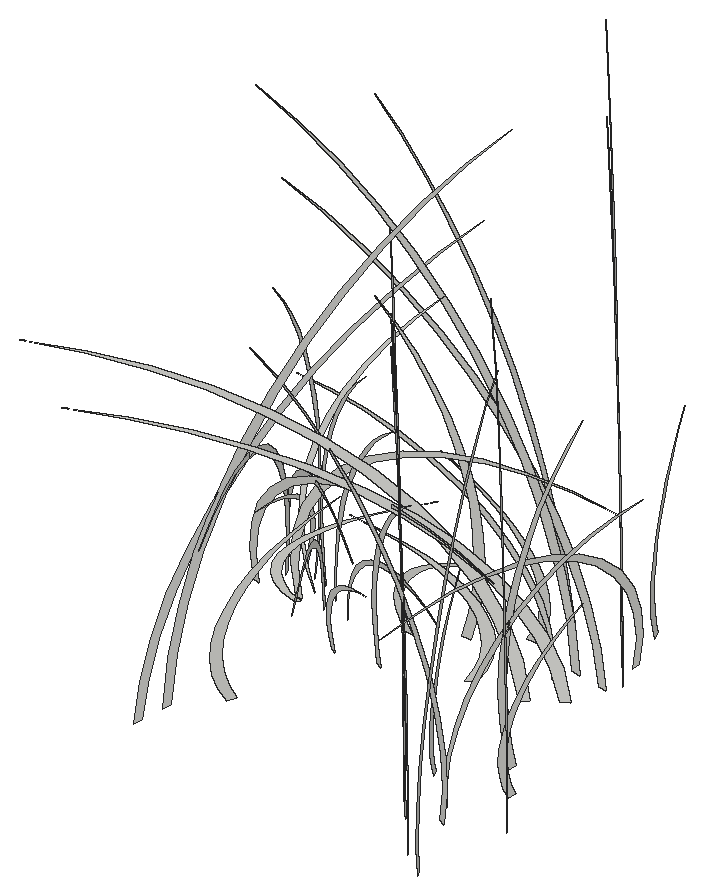
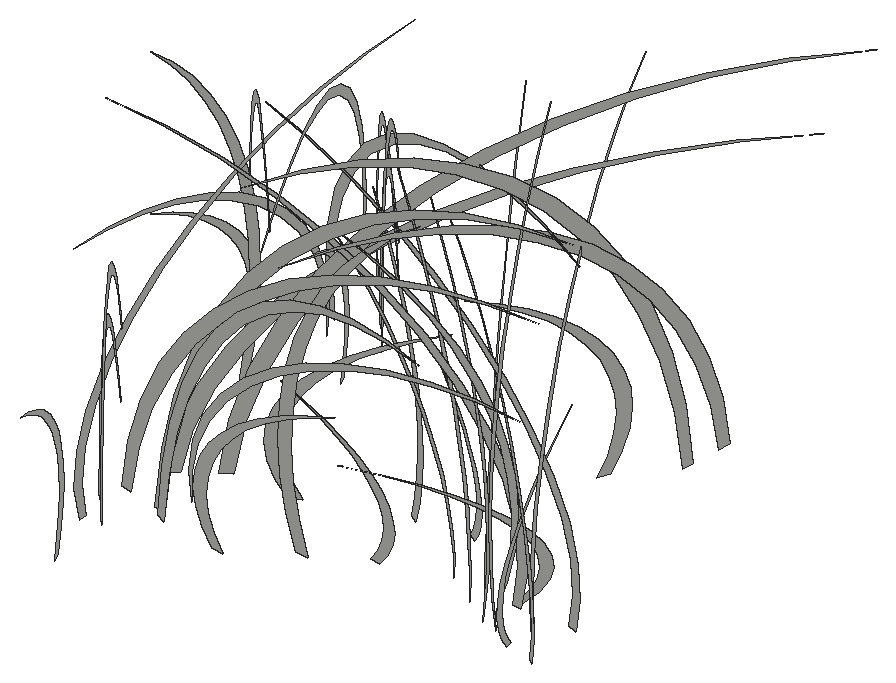
# SketchUp Ruby script. Lengths in inches.
U = 1.inch
M = Sketchup.active_model
def pt(a) = Geom::Point3d.new(a.map { |v| v * U })
def face(e, loops, mat)
  f = e.add_face(loops[0].map { |a| pt(a) })
  loops[1..].each { |l| e.add_face(l.map { |a| pt(a) }).erase! }
  f.material = f.back_material = mat if mat
  f
end
# faces: each face lists its corners as indices into pts; further lists are holes
def faces(e, pts, list, mat = nil) = list.each { |f| face(e, (f[0].is_a?(Array) ? f : [f]).map { |l| l.map { |i| pts[i] } }, mat) }
# xy, xz, yz: faces in a plane at the given z, y or x. An outline is a flat list of corners, or four numbers for a rectangle; further outlines are holes
def ring(l) = l.size == 4 ? [[l[0], l[1]], [l[2], l[1]], [l[2], l[3]], [l[0], l[3]]] : l.each_slice(2).to_a
def flat(e, list, mat, &to3) = list.each { |f| face(e, (f[0].is_a?(Array) ? f : [f]).map { |l| ring(l).map { |u, v| to3.(u, v) } }, mat) }
def xy(e, z, list, mat = nil) = flat(e, list, mat) { |x, y| [x, y, z] }
def xz(e, y, list, mat = nil) = flat(e, list, mat) { |x, z| [x, y, z] }
def yz(e, x, list, mat = nil) = flat(e, list, mat) { |y, z| [x, y, z] }
def lines(e, pts, list) = list.each { |a, b| e.add_line(pt(pts[a]), pt(pts[b])) }
# prism: a flat outline (further loops are holes) pulled along v
def prism(e, loops, v, mat = nil)
  f = face(e, loops, mat); d = Geom::Vector3d.new(v.map { |x| x * U })
  f.pushpull(f.normal.samedirection?(d) ? d.length : -d.length)
end
def box(e, o, s, mat = nil) = prism(e, [[o, [o[0] + s[0], o[1], o[2]], [o[0] + s[0], o[1] + s[1], o[2]], [o[0], o[1] + s[1], o[2]]]], [0, 0, s[2]], mat)
def at(x, y, z, deg = 0) = Geom::Transformation.translation(pt([x, y, z])) * Geom::Transformation.rotation(ORIGIN, Z_AXIS, deg.degrees)
def axes(o, x, y, z) = Geom::Transformation.new([*x, 0, *y, 0, *z, 0, *pt(o).to_a, 1])
def part(name) = M.definitions.add(name)
# library, detail: a bought-in or finely detailed component or shape, given as its bounding box
def library(name, o, s) = part(name).tap { |d| box(d.entities, o, s) }
def detail(e, o, s) = box(e.add_group.entities, o, s)
def put(e, d, t, mat = nil) = e.add_instance(d, t).tap { |i| i.material = mat if mat }
def group(e, t, mat = nil) = e.add_group.tap { |g| g.transformation = t; g.material = mat if mat }.entities
root = M.entities
g1 = group(root,at(61.625,583.2,0.02))
p = [[2.45,-7.42,6.49],[1.99,-6.01,6.08],[1.56,-4.73,5.625],[1.19,-3.6,5.14],[0.87,-2.64,4.62],[0.61,-1.83,4.08],
  [0.4,-1.21,3.52],[0.25,-0.76,2.9375],[0.16,-0.5,2.35],[0.14,-0.42,1.76],[0.18,-0.53,1.16],[0.28,-0.83,0.58],
  [0.43,-1.3125,0],[0.33,-0.99,0],[0.15,-0.44,0.57],[0.03,-0.1,1.16],[-0.02,0.05,1.75],[0.01,-0.02,2.35],
  [0.09,-0.28,2.94],[0.25,-0.76,3.53],[0.47,-1.43,4.1],[0.76,-2.29,4.64],[1.1,-3.33,5.16],[1.5,-4.54,5.65],
  [1.95,-5.91,6.09]]
faces(g1,p,[[0,1,2,3,4,5,6,7,8,9,10,11,12,13,14,15,16,17,18,19,20,21,22,23,24]])
g2 = group(root,at(62.74,582.29,0.02))
p = [[0.26,-0.74,0],[0.12,-0.33,1.62],[0.03,-0.08,3.26],[0,0,4.9],[0.03,-0.08,6.54],[0.11,-0.32,8.18],
  [0.26,-0.73,9.8],[0.46,-1.29,11.4],[0.71,-2.02,12.97],[1.03,-2.89,14.51],[1.39,-3.92,16],[1.8,-5.1,17.45],
  [2.27,-6.41,18.84],[1.83,-5.17,17.43],[1.44,-4.07,15.97],[1.09,-3.09,14.46],[0.8,-2.25,12.93],[0.55,-1.56,11.36],
  [0.35,-1,9.76],[0.21,-0.59,8.15],[0.12,-0.33,6.52],[0.07,-0.21,4.89],[0.08,-0.24,3.25],[0.15,-0.41,1.62]]
faces(g2,p,[[0,1,2,3,4,5,6,7,8,9,10,11,12,13,14,15,16,17,18,19,20,21,22,23]])
g3 = group(root,at(62.67,578.69,0.02))
p = [[6.35,4.55,5.51],[5.14,3.68,5.16],[4.05,2.9,4.78],[3.09,2.21,4.37],[2.26,1.62,3.93],[1.57,1.125,3.47],
  [1.03,0.74,2.99],[0.65,0.47,2.5],[0.43,0.31,2],[0.36,0.26,1.49],[0.46,0.33,0.99],[0.71,0.51,0.49],
  [1.125,0.8,0],[0.85,0.61,0],[0.38,0.27,0.48],[0.08,0.06,0.98],[-0.04,-0.03,1.49],[0.01,0.01,2],
  [0.24,0.17,2.5],[0.65,0.46,3],[1.22,0.875,3.48],[1.96,1.4,3.95],[2.85,2.04,4.39],[3.89,2.78,4.8],
  [5.0625,3.62,5.18]]
faces(g3,p,[[0,1,2,3,4,5,6,7,8,9,10,11,12,13,14,15,16,17,18,19,20,21,22,23,24]])
g4 = group(root,at(63.21,580.03,0.02))
p = [[0.625,0.47,0],[0.28,0.21,1.38],[0.07,0.05,2.77],[0,0,4.16],[0.07,0.05,5.5625],[0.28,0.21,6.95],
  [0.62,0.46,8.33],[1.1,0.82,9.69],[1.71,1.28,11.03],[2.46,1.84,12.33],[3.33,2.49,13.6],[4.33,3.24,14.83],
  [5.45,4.07,16.01],[4.4,3.29,14.8125],[3.46,2.58,13.57],[2.63,1.96,12.3],[1.92,1.43,10.99],[1.32,0.99,9.65],
  [0.85,0.64,8.3],[0.5,0.375,6.93],[0.28,0.21,5.55],[0.18,0.13,4.16],[0.2,0.15,2.77],[0.35,0.26,1.38]]
faces(g4,p,[[0,1,2,3,4,5,6,7,8,9,10,11,12,13,14,15,16,17,18,19,20,21,22,23]])
g5 = group(root,at(65.02,565.47,0.02))
p = [[1.63,20.71,16.73],[1.875,23.84,17.17],[1.64,20.8125,16.64],[1.41,17.89,15.9],[1.1875,15.1,14.96],[0.98,12.48,13.84],
  [0.79,10.06,12.54],[0.62,7.86,11.08],[0.47,5.91,9.48],[0.33,4.23,7.76],[0.22,2.84,5.92],[0.14,1.75,4.01],
  [0.08,0.98,2.02],[0.04,0.54,0],[0,0,0],[0.03,0.36,2.07],[0.09,1.09,4.1],[0.17,2.15,6.07],
  [0.28,3.55,7.94],[0.41,5.27,9.7],[0.57,7.28,11.33],[0.75,9.55,12.79],[0.95,12.07,14.08],[1.16,14.79,15.17],
  [1.39,17.68,16.0625]]
faces(g5,p,[[0,1,2,3,4,5,6,7,8,9,10,11,12,13,14,15,16,17,18,19,20,21,22,23,24]])
g6 = group(root,at(63.16,581.76,0.02))
p = [[0.65,-0.43,0],[0.29,-0.19,1.24],[0.07,-0.05,2.49],[0,0,3.75],[0.07,-0.05,5.01],[0.29,-0.1875,6.26],
  [0.65,-0.43,7.5],[1.15,-0.75,8.73],[1.79,-1.18,9.93],[2.57,-1.6875,11.11],[3.48,-2.29,12.25],[4.52,-2.97,13.36],
  [5.68,-3.74,14.43],[4.59,-3.02,13.35],[3.6,-2.37,12.23],[2.74,-1.8,11.08],[2,-1.3125,9.9],[1.38,-0.91,8.7],
  [0.89,-0.58,7.48],[0.52,-0.34,6.24],[0.29,-0.19,5],[0.18,-0.12,3.74],[0.21,-0.14,2.49],[0.37,-0.24,1.24]]
faces(g6,p,[[0,1,2,3,4,5,6,7,8,9,10,11,12,13,14,15,16,17,18,19,20,21,22,23]])
g7 = group(root,at(65.17,567.4,0.02))
p = [[1.63,20.71,20.75],[1.875,23.84,21.3],[1.64,20.8125,20.63],[1.41,17.89,19.72],[1.1875,15.1,18.55],[0.98,12.48,17.16],
  [0.79,10.06,15.55],[0.62,7.86,13.74],[0.47,5.91,11.76],[0.33,4.23,9.62],[0.22,2.84,7.35],[0.14,1.75,4.97],
  [0.08,0.98,2.51],[0.04,0.54,0],[0,0,0],[0.03,0.36,2.57],[0.09,1.09,5.09],[0.17,2.15,7.53],
  [0.28,3.55,9.85],[0.41,5.27,12.03],[0.57,7.28,14.04],[0.75,9.55,15.86],[0.95,12.07,17.46],[1.16,14.79,18.82],
  [1.39,17.68,19.92]]
faces(g7,p,[[0,1,2,3,4,5,6,7,8,9,10,11,12,13,14,15,16,17,18,19,20,21,22,23,24]])
g8 = group(root,at(61.36,581.64,0.02))
p = [[0.35,-0.68,0],[0.16,-0.3,0],[0,0,1.7],[0.0625,-0.12,3.4],[0.34,-0.66,5.07],[0.83,-1.61,6.67],
  [1.52,-2.93,8.15],[2.39,-4.61,9.48],[3.42,-6.59,10.63],[4.58,-8.84,11.57],[5.85,-11.28,12.27],[7.1875,-13.87,12.71],
  [8.57,-16.53,12.89],[9.96,-19.21,12.81],[8.6,-16.58,12.82],[7.25,-13.98,12.59],[5.95,-11.47,12.1],[4.72,-9.1,11.38],
  [3.59,-6.93,10.4375],[2.6,-5.01,9.3],[1.75,-3.38,7.99],[1.08,-2.09,6.53],[0.6,-1.15,4.97],[0.31,-0.6,3.33],
  [0.23,-0.4375,1.67]]
faces(g8,p,[[0,1,2,3,4,5,6,7,8,9,10,11,12,13,14,15,16,17,18,19,20,21,22,23,24]])
g9 = group(root,at(78.42,582.08,0.02))
p = [[-20.32,4.32,20.75],[-23.39,4.97,21.3],[-20.42,4.34,20.63],[-17.55,3.73,19.72],[-14.82,3.15,18.55],[-12.25,2.6,17.16],
  [-9.87,2.1,15.55],[-7.71,1.64,13.74],[-5.8,1.23,11.76],[-4.15,0.88,9.62],[-2.79,0.59,7.35],[-1.72,0.37,4.97],
  [-0.96,0.21,2.51],[-0.53,0.11,0],[0,0,0],[-0.36,0.08,2.57],[-1.07,0.23,5.09],[-2.11,0.45,7.53],
  [-3.49,0.74,9.85],[-5.17,1.1,12.03],[-7.14,1.52,14.04],[-9.375,1.99,15.86],[-11.84,2.52,17.46],[-14.51,3.08,18.82],
  [-17.35,3.6875,19.92]]
faces(g9,p,[[0,1,2,3,4,5,6,7,8,9,10,11,12,13,14,15,16,17,18,19,20,21,22,23,24]])
g10 = group(root,at(60.26,582.81,0.02))
p = [[0.47,-0.41,0],[0.21,-0.18,0],[0,0,1.2],[0.08,-0.07,2.41],[0.46,-0.4,3.6],[1.12,-0.98,4.74],
  [2.04,-1.79,5.79],[3.2,-2.8125,6.73],[4.58,-4.02,7.55],[6.13,-5.39,8.21],[7.83,-6.875,8.71],[9.62,-8.45,9.03],
  [11.47,-10.08,9.16],[13.33,-11.71,9.09],[11.51,-10.11,9.11],[9.7,-8.52,8.9375],[7.96,-6.99,8.59],[6.31,-5.55,8.08],
  [4.81,-4.22,7.41],[3.48,-3.05,6.6],[2.35,-2.0625,5.67],[1.45,-1.27,4.64],[0.8,-0.7,3.53],[0.41,-0.36,2.37],
  [0.3,-0.27,1.18]]
faces(g10,p,[[0,1,2,3,4,5,6,7,8,9,10,11,12,13,14,15,16,17,18,19,20,21,22,23,24]])
g11 = group(root,at(60.26,582.81,0.02))
p = [[0.47,-0.41,0],[0.21,-0.18,0],[0,0,1.2],[0.08,-0.07,2.41],[0.46,-0.4,3.6],[1.12,-0.98,4.74],
  [2.04,-1.79,5.79],[3.2,-2.8125,6.73],[4.58,-4.02,7.55],[6.13,-5.39,8.21],[7.83,-6.875,8.71],[9.62,-8.45,9.03],
  [11.47,-10.08,9.16],[13.33,-11.71,9.09],[11.51,-10.11,9.11],[9.7,-8.52,8.9375],[7.96,-6.99,8.59],[6.31,-5.55,8.08],
  [4.81,-4.22,7.41],[3.48,-3.05,6.6],[2.35,-2.0625,5.67],[1.45,-1.27,4.64],[0.8,-0.7,3.53],[0.41,-0.36,2.37],
  [0.3,-0.27,1.18]]
faces(g11,p,[[0,1,2,3,4,5,6,7,8,9,10,11,12,13,14,15,16,17,18,19,20,21,22,23,24]])
g12 = group(root,at(77.95,582.5,0.02))
p = [[-18.35,9.75,18.05],[-21.11,11.23,18.53],[-18.43,9.8,17.95],[-15.84,8.42,17.15],[-13.375,7.11,16.14],[-11.05,5.88,14.93],
  [-8.91,4.74,13.53],[-6.96,3.7,11.96],[-5.23,2.78,10.23],[-3.75,1.99,8.37],[-2.51,1.34,6.39],[-1.55,0.83,4.32],
  [-0.87,0.46,2.18],[-0.48,0.25,0],[0,0,0],[-0.32,0.17,2.23],[-0.96,0.51,4.43],[-1.91,1.01,6.55],
  [-3.15,1.67,8.57],[-4.67,2.48,10.47],[-6.45,3.43,12.22],[-8.46,4.5,13.8],[-10.6875,5.68,15.1875],[-13.1,6.97,16.37],
  [-15.66,8.33,17.33]]
faces(g12,p,[[0,1,2,3,4,5,6,7,8,9,10,11,12,13,14,15,16,17,18,19,20,21,22,23,24]])
g13 = group(root,at(66.72,568.99,0.02))
p = [[2.34,6.79,9.0625],[1.91,5.55,8.49],[1.52,4.43,7.85],[1.18,3.44,7.18],[0.89,2.58,6.45],[0.65,1.88,5.7],
  [0.46,1.33,4.91],[0.32,0.93,4.1],[0.24,0.7,3.28],[0.22,0.64,2.45],[0.25,0.74,1.625],[0.34,1,0.8],
  [0.49,1.42,0],[0.3,0.875,0],[0.14,0.4,0.81],[0.04,0.11,1.65],[0,0,2.49],[0.03,0.07,3.34],
  [0.11,0.33,4.17],[0.27,0.77,4.99],[0.48,1.38,5.79],[0.75,2.17,6.54],[1.07,3.11,7.26],[1.45,4.2,7.92],
  [1.87,5.43,8.52]]
faces(g13,p,[[0,1,2,3,4,5,6,7,8,9,10,11,12,13,14,15,16,17,18,19,20,21,22,23,24]])
g14 = group(root,at(78.15,578.71,0.02))
p = [[-17.04,-11.89,18.05],[-19.61,-13.68,18.53],[-17.12,-11.94,17.95],[-14.72,-10.27,17.15],[-12.42,-8.67,16.14],[-10.27,-7.16,14.93],
  [-8.28,-5.77,13.53],[-6.47,-4.51,11.96],[-4.86,-3.39,10.23],[-3.48,-2.43,8.37],[-2.34,-1.63,6.39],[-1.44,-1.01,4.32],
  [-0.81,-0.5625,2.18],[-0.44,-0.31,0],[0,0,0],[-0.3,-0.21,2.23],[-0.89,-0.62,4.43],[-1.77,-1.24,6.55],
  [-2.92,-2.04,8.57],[-4.33,-3.02,10.47],[-5.99,-4.18,12.22],[-7.86,-5.48,13.8],[-9.93,-6.93,15.1875],[-12.17,-8.49,16.37],
  [-14.55,-10.15,17.33]]
faces(g14,p,[[0,1,2,3,4,5,6,7,8,9,10,11,12,13,14,15,16,17,18,19,20,21,22,23,24]])
g15 = group(root,at(80.31,581.68,0.02))
p = [[-20.32,4.32,16.73],[-23.39,4.97,17.17],[-20.42,4.34,16.64],[-17.55,3.73,15.9],[-14.82,3.15,14.96],[-12.25,2.6,13.84],
  [-9.87,2.1,12.54],[-7.71,1.64,11.08],[-5.8,1.23,9.48],[-4.15,0.88,7.76],[-2.79,0.59,5.92],[-1.72,0.37,4.01],
  [-0.96,0.21,2.02],[-0.53,0.11,0],[0,0,0],[-0.36,0.08,2.07],[-1.07,0.23,4.1],[-2.11,0.45,6.07],
  [-3.49,0.74,7.94],[-5.17,1.1,9.7],[-7.14,1.52,11.33],[-9.375,1.99,12.79],[-11.84,2.52,14.08],[-14.51,3.08,15.17],
  [-17.35,3.6875,16.0625]]
faces(g15,p,[[0,1,2,3,4,5,6,7,8,9,10,11,12,13,14,15,16,17,18,19,20,21,22,23,24]])
g16 = group(root,at(64.98,580.56,0.02))
p = [[7.3,-4.8,13.72],[6.14,-4.04,12.71],[5.07,-3.33,11.66],[4.1,-2.69,10.58],[3.22,-2.12,9.48],[2.46,-1.61,8.34],
  [1.79,-1.18,7.19],[1.23,-0.8125,6.02],[0.79,-0.52,4.83],[0.45,-0.29,3.63],[0.22,-0.14,2.43],[0.1,-0.07,1.21],
  [0.1,-0.0625,0],[0,0,1.22],[0.04,-0.02,2.44],[0.2,-0.13,3.66],[0.5,-0.33,4.87],[0.92,-0.61,6.07],
  [1.47,-0.97,7.25],[2.15,-1.41,8.41],[2.95,-1.9375,9.54],[3.87,-2.54,10.64],[4.9,-3.22,11.71],[6.05,-3.98,12.73]]
faces(g16,p,[[0,1,2,3,4,5,6,7,8,9,10,11,12,13,14,15,16,17,18,19,20,21,22,23]])
g17 = group(root,at(77.73,581,0.02))
p = [[-16.72,1.64,9.9],[-14.47,1.42,9.83],[-12.26,1.2,9.59],[-10.125,0.99,9.18],[-8.11,0.8,8.61],[-6.26,0.61,7.88],
  [-4.6,0.45,7.02],[-3.17,0.31,6.03],[-1.98,0.19,4.95],[-1.08,0.11,3.78],[-0.46,0.05,2.55],[-0.15,0.01,1.28],
  [-0.15,0.01,0],[0,0,1.3],[-0.2,0.02,2.61],[-0.73,0.07,3.875],[-1.6,0.16,5.09],[-2.77,0.27,6.21],
  [-4.23,0.41,7.22],[-5.93,0.58,8.1],[-7.85,0.77,8.82],[-9.93,0.97,9.37],[-12.14,1.19,9.74],[-14.42,1.41,9.92]]
faces(g17,p,[[0,1,2,3,4,5,6,7,8,9,10,11,12,13,14,15,16,17,18,19,20,21,22,23]])
g18 = group(root,at(67.12,577.25,0.02))
p = [[4.9375,-3.25,5.51],[4.03,-2.65,5.16],[3.22,-2.12,4.78],[2.5,-1.64,4.37],[1.88,-1.24,3.93],[1.37,-0.9,3.47],
  [0.97,-0.63,2.99],[0.68,-0.45,2.5],[0.51,-0.34,2],[0.46,-0.3,1.49],[0.53,-0.35,0.99],[0.73,-0.48,0.49],
  [1.03,-0.68,0],[0.64,-0.42,0],[0.29,-0.19,0.5],[0.08,-0.05,1],[0,0,1.52],[0.05,-0.04,2.03],
  [0.24,-0.16,2.54],[0.56,-0.37,3.04],[1.01,-0.66,3.52],[1.58,-1.04,3.98],[2.26,-1.49,4.42],[3.06,-2.01,4.82],
  [3.95,-2.6,5.1875]]
faces(g18,p,[[0,1,2,3,4,5,6,7,8,9,10,11,12,13,14,15,16,17,18,19,20,21,22,23,24]])
g19 = group(root,at(73.23,581.44,0.02))
p = [[-7.14,0.7,16.02],[-5.84,0.57,15.01],[-4.66,0.46,13.89],[-3.62,0.35,12.69],[-2.72,0.27,11.42],[-1.98,0.19,10.08],
  [-1.4,0.14,8.6875],[-0.98,0.1,7.26],[-0.74,0.07,5.8],[-0.67,0.07,4.34],[-0.77,0.08,2.87],[-1.05,0.1,1.42],
  [-1.5,0.15,0],[-0.92,0.09,0],[-0.42,0.04,1.44],[-0.12,0.01,2.92],[0,0,4.41],[-0.08,0.01,5.9],
  [-0.35,0.03,7.38],[-0.8125,0.08,8.83],[-1.46,0.14,10.23],[-2.28,0.22,11.57],[-3.27,0.32,12.83],[-4.42,0.43,14.01],
  [-5.72,0.5625,15.07]]
faces(g19,p,[[0,1,2,3,4,5,6,7,8,9,10,11,12,13,14,15,16,17,18,19,20,21,22,23,24]])
g20 = group(root,at(73.23,581.44,0.02))
p = [[-7.14,0.7,16.02],[-5.84,0.57,15.01],[-4.66,0.46,13.89],[-3.62,0.35,12.69],[-2.72,0.27,11.42],[-1.98,0.19,10.08],
  [-1.4,0.14,8.6875],[-0.98,0.1,7.26],[-0.74,0.07,5.8],[-0.67,0.07,4.34],[-0.77,0.08,2.87],[-1.05,0.1,1.42],
  [-1.5,0.15,0],[-0.92,0.09,0],[-0.42,0.04,1.44],[-0.12,0.01,2.92],[0,0,4.41],[-0.08,0.01,5.9],
  [-0.35,0.03,7.38],[-0.8125,0.08,8.83],[-1.46,0.14,10.23],[-2.28,0.22,11.57],[-3.27,0.32,12.83],[-4.42,0.43,14.01],
  [-5.72,0.5625,15.07]]
faces(g20,p,[[0,1,2,3,4,5,6,7,8,9,10,11,12,13,14,15,16,17,18,19,20,21,22,23,24]])
g21 = group(root,at(79.73,579.8125,0.02))
p = [[-17.04,-11.89,14.56],[-19.61,-13.68,14.94],[-17.12,-11.94,14.48],[-14.72,-10.27,13.83],[-12.42,-8.67,13.02],[-10.27,-7.16,12.04],
  [-8.28,-5.77,10.91],[-6.47,-4.51,9.64],[-4.86,-3.39,8.25],[-3.48,-2.43,6.75],[-2.34,-1.63,5.15],[-1.44,-1.01,3.49],
  [-0.81,-0.5625,1.76],[-0.44,-0.31,0],[0,0,0],[-0.3,-0.21,1.8],[-0.89,-0.62,3.57],[-1.77,-1.24,5.28],
  [-2.92,-2.04,6.91],[-4.33,-3.02,8.44],[-5.99,-4.18,9.85],[-7.86,-5.48,11.13],[-9.93,-6.93,12.25],[-12.17,-8.49,13.2],
  [-14.55,-10.15,13.97]]
faces(g21,p,[[0,1,2,3,4,5,6,7,8,9,10,11,12,13,14,15,16,17,18,19,20,21,22,23,24]])
g22 = group(root,at(64.92,579.83,0.02))
p = [[9.63,-14.13,10.18],[11.08,-16.26,10.45],[9.68,-14.2,10.13],[8.32,-12.2,9.68],[7.02,-10.3,9.11],[5.8,-8.51,8.42],
  [4.68,-6.86,7.63],[3.65,-5.36,6.75],[2.75,-4.03,5.77],[1.97,-2.89,4.72],[1.32,-1.9375,3.61],[0.81,-1.2,2.4375],
  [0.46,-0.67,1.23],[0.25,-0.37,0],[0,0,0],[0.17,-0.25,1.26],[0.5,-0.74,2.5],[1,-1.47,3.69],
  [1.65,-2.42,4.83],[2.45,-3.59,5.91],[3.38,-4.96,6.89],[4.44,-6.52,7.78],[5.61,-8.23,8.57],[6.88,-10.09,9.24],
  [8.22,-12.0625,9.78]]
faces(g22,p,[[0,1,2,3,4,5,6,7,8,9,10,11,12,13,14,15,16,17,18,19,20,21,22,23,24]])
g23 = group(root,at(60.38,579.93,0.02))
p = [[0.76,-0.3,0],[0.34,-0.14,0],[0,0,1.44],[0.14,-0.05,2.89],[0.74,-0.3,4.3125],[1.8,-0.72,5.67],
  [3.29,-1.32,6.93],[5.17,-2.08,8.0625],[7.4,-2.97,9.04],[9.91,-3.98,9.83],[12.66,-5.09,10.43],[15.56,-6.25,10.81],
  [18.55,-7.46,10.96],[21.55,-8.66,10.89],[18.6,-7.48,10.9],[15.6875,-6.31,10.7],[12.87,-5.17,10.29],[10.21,-4.1,9.67],
  [7.78,-3.125,8.875],[5.62,-2.26,7.9],[3.79,-1.53,6.79],[2.34,-0.94,5.55],[1.29,-0.52,4.22],[0.67,-0.27,2.83],
  [0.49,-0.2,1.42]]
faces(g23,p,[[0,1,2,3,4,5,6,7,8,9,10,11,12,13,14,15,16,17,18,19,20,21,22,23,24]])
g24 = group(root,at(68.66,580.38,0.02))
p = [[5.86,-0.75,5.51],[4.79,-0.62,5.16],[3.82,-0.49,4.78],[2.97,-0.38,4.37],[2.23,-0.29,3.93],[1.62,-0.21,3.47],
  [1.15,-0.15,2.99],[0.81,-0.1,2.5],[0.61,-0.08,2],[0.55,-0.07,1.49],[0.63,-0.08,0.99],[0.86,-0.11,0.49],
  [1.23,-0.16,0],[0.75,-0.1,0],[0.35,-0.04,0.5],[0.09,-0.01,1],[0,0,1.52],[0.0625,-0.01,2.03],
  [0.29,-0.04,2.54],[0.67,-0.09,3.04],[1.19,-0.15,3.52],[1.87,-0.24,3.98],[2.68,-0.34,4.42],[3.63,-0.47,4.82],
  [4.69,-0.6,5.1875]]
faces(g24,p,[[0,1,2,3,4,5,6,7,8,9,10,11,12,13,14,15,16,17,18,19,20,21,22,23,24]])
g25 = group(root,at(79.45,583.95,0.02))
p = [[-13.49,15.8,20.75],[-15.53,18.18,21.3],[-13.56,15.875,20.63],[-11.65,13.64,19.72],[-9.84,11.52,18.55],[-8.13,9.52,17.16],
  [-6.55,7.67,15.55],[-5.12,6,13.74],[-3.85,4.51,11.76],[-2.76,3.23,9.62],[-1.85,2.17,7.35],[-1.14,1.34,4.97],
  [-0.64,0.75,2.51],[-0.35,0.41,0],[0,0,0],[-0.24,0.28,2.57],[-0.71,0.83,5.09],[-1.4,1.64,7.53],
  [-2.31,2.71,9.85],[-3.43,4.02,12.03],[-4.74,5.55,14.04],[-6.22,7.29,15.86],[-7.86,9.21,17.46],[-9.64,11.28,18.82],
  [-11.52,13.49,19.92]]
faces(g25,p,[[0,1,2,3,4,5,6,7,8,9,10,11,12,13,14,15,16,17,18,19,20,21,22,23,24]])
g26 = group(root,at(69.66,577.49,0.02))
p = [[4.9375,-3.25,11.21],[4.03,-2.65,10.5],[3.22,-2.12,9.72],[2.5,-1.64,8.88],[1.88,-1.24,7.99],[1.37,-0.9,7.05],
  [0.97,-0.63,6.08],[0.68,-0.45,5.08],[0.51,-0.34,4.06],[0.46,-0.3,3.03],[0.53,-0.35,2.01],[0.73,-0.48,1],
  [1.03,-0.68,0],[0.64,-0.42,0],[0.29,-0.19,1.01],[0.08,-0.05,2.04],[0,0,3.08],[0.05,-0.04,4.13],
  [0.24,-0.16,5.16],[0.56,-0.37,6.18],[1.01,-0.66,7.16],[1.58,-1.04,8.1],[2.26,-1.49,8.98],[3.06,-2.01,9.8],
  [3.95,-2.6,10.54]]
faces(g26,p,[[0,1,2,3,4,5,6,7,8,9,10,11,12,13,14,15,16,17,18,19,20,21,22,23,24]])
g27 = group(root,at(75.82,583.13,0.02))
p = [[-7.14,0.7,7.88],[-5.84,0.57,7.38],[-4.66,0.46,6.83],[-3.62,0.35,6.24],[-2.72,0.27,5.62],[-1.98,0.19,4.96],
  [-1.4,0.14,4.27],[-0.98,0.1,3.57],[-0.74,0.07,2.86],[-0.67,0.07,2.13],[-0.77,0.08,1.41],[-1.05,0.1,0.7],
  [-1.5,0.15,0],[-0.92,0.09,0],[-0.42,0.04,0.71],[-0.12,0.01,1.43],[0,0,2.17],[-0.08,0.01,2.9],
  [-0.35,0.03,3.63],[-0.8125,0.08,4.34],[-1.46,0.14,5.03],[-2.28,0.22,5.69],[-3.27,0.32,6.3125],[-4.42,0.43,6.89],
  [-5.72,0.5625,7.41]]
faces(g27,p,[[0,1,2,3,4,5,6,7,8,9,10,11,12,13,14,15,16,17,18,19,20,21,22,23,24]])
g28 = group(root,at(66.55,579.53,0.02))
p = [[11.55,-7.59,6.92],[10,-6.57,6.88],[8.47,-5.57,6.71],[7,-4.6,6.42],[5.61,-3.6875,6.02],[4.33,-2.84,5.51],
  [3.18,-2.09,4.91],[2.1875,-1.4375,4.22],[1.37,-0.9,3.46],[0.74,-0.49,2.64],[0.32,-0.21,1.78],[0.1,-0.07,0.89],
  [0.1,-0.07,0],[0,0,0.91],[0.14,-0.09,1.82],[0.51,-0.33,2.71],[1.1,-0.73,3.56],[1.91,-1.26,4.34],
  [2.92,-1.92,5.05],[4.1,-2.69,5.67],[5.42,-3.56,6.17],[6.86,-4.51,6.56],[8.39,-5.51,6.8125],[9.96,-6.55,6.9375]]
faces(g28,p,[[0,1,2,3,4,5,6,7,8,9,10,11,12,13,14,15,16,17,18,19,20,21,22,23]])
g29 = group(root,at(82.68,566.82,0.02))
p = [[-0.72,0.38,0],[-0.32,0.17,0],[0,0,1.82],[-0.13,0.07,3.66],[-0.71,0.375,5.45],[-1.72,0.91,7.17],
  [-3.14,1.67,8.77],[-4.93,2.62,10.2],[-7.05,3.75,11.43],[-9.45,5.02,12.4375],[-12.0625,6.41,13.1875],[-14.83,7.88,13.67],
  [-17.68,9.4,13.87],[-20.54,10.92,13.77],[-17.73,9.43,13.79],[-14.95,7.95,13.54],[-12.26,6.52,13.01],[-9.73,5.17,12.24],
  [-7.41,3.94,11.22],[-5.36,2.85,10],[-3.62,1.92,8.59],[-2.23,1.1875,7.02],[-1.23,0.65,5.34],[-0.64,0.34,3.59],
  [-0.47,0.25,1.79]]
faces(g29,p,[[0,1,2,3,4,5,6,7,8,9,10,11,12,13,14,15,16,17,18,19,20,21,22,23,24]])
g30 = group(root,at(75.93,578.88,0.02))
p = [[-6.73,-2.5,7.88],[-5.5,-2.04,7.38],[-4.39,-1.63,6.83],[-3.41,-1.27,6.24],[-2.5625,-0.95,5.62],[-1.86,-0.69,4.96],
  [-1.32,-0.49,4.27],[-0.93,-0.34,3.57],[-0.7,-0.26,2.86],[-0.63,-0.23,2.13],[-0.73,-0.27,1.41],[-0.99,-0.37,0.7],
  [-1.41,-0.52,0],[-0.87,-0.32,0],[-0.4,-0.15,0.71],[-0.11,-0.04,1.43],[0,0,2.17],[-0.07,-0.03,2.9],
  [-0.33,-0.12,3.63],[-0.76,-0.28,4.34],[-1.37,-0.51,5.03],[-2.15,-0.8,5.69],[-3.08,-1.15,6.3125],[-4.17,-1.55,6.89],
  [-5.39,-2,7.41]]
faces(g30,p,[[0,1,2,3,4,5,6,7,8,9,10,11,12,13,14,15,16,17,18,19,20,21,22,23,24]])
g31 = group(root,at(79.48,567.61,0.02))
p = [[-11.94,13.98,18.36],[-13.74,16.09,18.85],[-12,14.05,18.26],[-10.3125,12.07,17.45],[-8.71,10.19,16.42],[-7.2,8.43,15.1875],
  [-5.8,6.79,13.76],[-4.53,5.31,12.16],[-3.41,3.99,10.41],[-2.4375,2.86,8.51],[-1.64,1.92,6.5],[-1.01,1.18,4.4],
  [-0.57,0.66,2.22],[-0.3125,0.36,0],[0,0,0],[-0.21,0.25,2.27],[-0.625,0.73,4.5],[-1.24,1.45,6.66],
  [-2.05,2.4,8.72],[-3.04,3.56,10.65],[-4.2,4.91,12.43],[-5.51,6.45,14.04],[-6.96,8.15,15.45],[-8.53,9.98,16.65],
  [-10.2,11.9375,17.625]]
faces(g31,p,[[0,1,2,3,4,5,6,7,8,9,10,11,12,13,14,15,16,17,18,19,20,21,22,23,24]])
g32 = group(root,at(80.7,582.48,0.02))
p = [[-13.49,15.8,16.73],[-15.53,18.18,17.17],[-13.56,15.875,16.64],[-11.65,13.64,15.9],[-9.84,11.52,14.96],[-8.13,9.52,13.84],
  [-6.55,7.67,12.54],[-5.12,6,11.08],[-3.85,4.51,9.48],[-2.76,3.23,7.76],[-1.85,2.17,5.92],[-1.14,1.34,4.01],
  [-0.64,0.75,2.02],[-0.35,0.41,0],[0,0,0],[-0.24,0.28,2.07],[-0.71,0.83,4.1],[-1.4,1.64,6.07],
  [-2.31,2.71,7.94],[-3.43,4.02,9.7],[-4.74,5.55,11.33],[-6.22,7.29,12.79],[-7.86,9.21,14.08],[-9.64,11.28,15.17],
  [-11.52,13.49,16.0625]]
faces(g32,p,[[0,1,2,3,4,5,6,7,8,9,10,11,12,13,14,15,16,17,18,19,20,21,22,23,24]])
g33 = group(root,at(80.59,566.31,0.02))
p = [[-11.94,13.98,14.81],[-13.74,16.09,15.2],[-12,14.05,14.73],[-10.3125,12.07,14.07],[-8.71,10.19,13.24],[-7.2,8.43,12.25],
  [-5.8,6.79,11.1],[-4.53,5.31,9.81],[-3.41,3.99,8.39],[-2.4375,2.86,6.86],[-1.64,1.92,5.24],[-1.01,1.18,3.55],
  [-0.57,0.66,1.79],[-0.3125,0.36,0],[0,0,0],[-0.21,0.25,1.83],[-0.625,0.73,3.63],[-1.24,1.45,5.37],
  [-2.05,2.4,7.03],[-3.04,3.56,8.59],[-4.2,4.91,10.02],[-5.51,6.45,11.32],[-6.96,8.15,12.46],[-8.53,9.98,13.43],
  [-10.2,11.9375,14.21]]
faces(g33,p,[[0,1,2,3,4,5,6,7,8,9,10,11,12,13,14,15,16,17,18,19,20,21,22,23,24]])
g34 = group(root,at(62.98,579.73,0.02))
p = [[0.76,-0.08,0],[0.34,-0.04,0],[0,0,1.7],[0.14,-0.02,3.4],[0.74,-0.08,5.07],[1.8,-0.2,6.67],
  [3.29,-0.36,8.15],[5.16,-0.57,9.48],[7.38,-0.82,10.63],[9.89,-1.09,11.57],[12.63,-1.39,12.27],[15.52,-1.71,12.71],
  [18.51,-2.04,12.89],[21.5,-2.375,12.81],[18.5625,-2.05,12.82],[15.65,-1.73,12.59],[12.84,-1.42,12.1],[10.1875,-1.125,11.38],
  [7.76,-0.86,10.4375],[5.61,-0.62,9.3],[3.79,-0.42,7.99],[2.33,-0.26,6.53],[1.29,-0.14,4.97],[0.67,-0.07,3.33],
  [0.49,-0.05,1.67]]
faces(g34,p,[[0,1,2,3,4,5,6,7,8,9,10,11,12,13,14,15,16,17,18,19,20,21,22,23,24]])
g35 = group(root,at(62.98,579.73,0.02))
p = [[0.76,-0.08,0],[0.34,-0.04,0],[0,0,1.7],[0.14,-0.02,3.4],[0.74,-0.08,5.07],[1.8,-0.2,6.67],
  [3.29,-0.36,8.15],[5.16,-0.57,9.48],[7.38,-0.82,10.63],[9.89,-1.09,11.57],[12.63,-1.39,12.27],[15.52,-1.71,12.71],
  [18.51,-2.04,12.89],[21.5,-2.375,12.81],[18.5625,-2.05,12.82],[15.65,-1.73,12.59],[12.84,-1.42,12.1],[10.1875,-1.125,11.38],
  [7.76,-0.86,10.4375],[5.61,-0.62,9.3],[3.79,-0.42,7.99],[2.33,-0.26,6.53],[1.29,-0.14,4.97],[0.67,-0.07,3.33],
  [0.49,-0.05,1.67]]
faces(g35,p,[[0,1,2,3,4,5,6,7,8,9,10,11,12,13,14,15,16,17,18,19,20,21,22,23,24]])
g36 = group(root,at(83.0625,563.41,0.02))
p = [[-0.57,0.67,0],[-0.25,0.3,0],[0,0,1.78],[-0.1,0.12,3.57],[-0.56,0.65,5.33],[-1.36,1.59,7.01],
  [-2.48,2.9,8.56],[-3.89,4.56,9.96],[-5.57,6.52,11.17],[-7.46,8.74,12.15],[-9.52,11.15,12.89],[-11.71,13.71,13.36],
  [-13.96,16.34,13.55],[-16.22,18.99,13.46],[-14,16.39,13.47],[-11.81,13.82,13.22],[-9.68,11.34,12.71],[-7.68,9,11.96],
  [-5.85,6.85,10.97],[-4.23,4.95,9.77],[-2.86,3.34,8.39],[-1.76,2.0625,6.86],[-0.97,1.14,5.22],[-0.5,0.59,3.5],
  [-0.37,0.43,1.75]]
faces(g36,p,[[0,1,2,3,4,5,6,7,8,9,10,11,12,13,14,15,16,17,18,19,20,21,22,23,24]])
g37 = group(root,at(79.41,586.17,0.02))
p = [[-3.15,6.45,9.0625],[-2.57,5.27,8.49],[-2.05,4.21,7.85],[-1.59,3.27,7.18],[-1.2,2.46,6.45],[-0.87,1.79,5.7],
  [-0.62,1.26,4.91],[-0.43,0.89,4.1],[-0.33,0.67,3.28],[-0.3,0.61,2.45],[-0.34,0.7,1.625],[-0.46,0.95,0.8],
  [-0.66,1.35,0],[-0.41,0.83,0],[-0.1875,0.38,0.81],[-0.05,0.1,1.65],[0,0,2.49],[-0.03,0.07,3.34],
  [-0.15,0.32,4.17],[-0.36,0.73,4.99],[-0.64,1.32,5.79],[-1,2.06,6.54],[-1.44,2.96,7.26],[-1.95,3.99,7.92],
  [-2.52,5.16,8.52]]
faces(g37,p,[[0,1,2,3,4,5,6,7,8,9,10,11,12,13,14,15,16,17,18,19,20,21,22,23,24]])
g38 = group(root,at(85.41,567.9,0.02))
p = [[-0.53,0.62,0],[-0.24,0.28,0],[0,0,2.1],[-0.1,0.11,4.2],[-0.52,0.61,6.27],[-1.26,1.48,8.24],
  [-2.31,2.7,10.08],[-3.625,4.25,11.72],[-5.1875,6.07,13.14],[-6.95,8.14,14.3],[-8.87,10.39,15.16],[-10.91,12.77,15.71],
  [-13,15.22,15.9375],[-15.11,17.6875,15.83],[-13.04,15.27,15.85],[-11,12.88,15.56],[-9.02,10.5625,14.96],[-7.16,8.38,14.07],
  [-5.45,6.38,12.9],[-3.94,4.61,11.49],[-2.66,3.11,9.87],[-1.64,1.92,8.07],[-0.9,1.06,6.14],[-0.47,0.55,4.12],
  [-0.34,0.4,2.06]]
faces(g38,p,[[0,1,2,3,4,5,6,7,8,9,10,11,12,13,14,15,16,17,18,19,20,21,22,23,24]])
g39 = group(root,at(79.44,569.57,0.02))
p = [[-2.79,5.71,8.02],[-2.28,4.67,7.51],[-1.82,3.72,6.95],[-1.41,2.89,6.35],[-1.06,2.17,5.71],[-0.77,1.58,5.04],
  [-0.54,1.12,4.35],[-0.38,0.79,3.63],[-0.29,0.59,2.9],[-0.26,0.54,2.17],[-0.3,0.62,1.4375],[-0.41,0.84,0.71],
  [-0.58,1.19,0],[-0.36,0.74,0],[-0.16,0.34,0.72],[-0.04,0.09,1.46],[0,0,2.21],[-0.03,0.0625,2.95],
  [-0.14,0.28,3.69],[-0.32,0.65,4.42],[-0.57,1.16,5.12],[-0.89,1.82,5.79],[-1.28,2.62,6.42],[-1.72,3.54,7.01],
  [-2.23,4.57,7.54]]
faces(g39,p,[[0,1,2,3,4,5,6,7,8,9,10,11,12,13,14,15,16,17,18,19,20,21,22,23,24]])
g40 = group(root,at(84.64,562.06,0.02))
p = [[-0.4375,0.76,0],[-0.19,0.34,0],[0,0,1.78],[-0.08,0.14,3.57],[-0.43,0.75,5.33],[-1.04,1.8125,7.01],
  [-1.9,3.31,8.56],[-2.99,5.2,9.96],[-4.27,7.43,11.17],[-5.73,9.96,12.15],[-7.3125,12.71,12.89],[-8.99,15.63,13.36],
  [-10.71,18.63,13.55],[-12.45,21.65,13.46],[-10.75,18.6875,13.47],[-9.0625,15.76,13.22],[-7.43,12.93,12.71],[-5.9,10.26,11.96],
  [-4.49,7.8125,10.97],[-3.25,5.65,9.77],[-2.19,3.8125,8.39],[-1.35,2.35,6.86],[-0.74,1.3,5.22],[-0.39,0.67,3.5],
  [-0.28,0.49,1.75]]
faces(g40,p,[[0,1,2,3,4,5,6,7,8,9,10,11,12,13,14,15,16,17,18,19,20,21,22,23,24]])
g41 = group(root,at(79.91,584.93,0.02))
p = [[0.05,-0.76,0],[0.02,-0.34,0],[0,0,1.46],[0.01,-0.14,2.93],[0.05,-0.74,4.375],[0.12,-1.8,5.75],
  [0.21,-3.29,7.03],[0.33,-5.16,8.18],[0.48,-7.38,9.17],[0.64,-9.9,9.98],[0.82,-12.63,10.58],[1,-15.53,10.97],
  [1.2,-18.51,11.125],[1.39,-21.51,11.05],[1.2,-18.57,11.0625],[1.01,-15.66,10.86],[0.83,-12.84,10.44],[0.66,-10.19,9.82],
  [0.5,-7.76,9.01],[0.36,-5.61,8.02],[0.24,-3.79,6.89],[0.15,-2.34,5.64],[0.08,-1.29,4.29],[0.04,-0.67,2.88],
  [0.03,-0.49,1.4375]]
faces(g41,p,[[0,1,2,3,4,5,6,7,8,9,10,11,12,13,14,15,16,17,18,19,20,21,22,23,24]])
g42 = group(root,at(81.46,568.18,0.02))
yz(g42,0,[[0.13,0,0,1.33,0.17,2.65,0.65,3.94,1.42,5.17,2.46,6.32,3.76,7.35,5.27,8.24,6.98,8.97,8.83,9.53,10.79,9.91,12.82,10.09,14.86,10.07,12.87,10,10.9,9.76,9,9.34,7.22,8.76,5.57,8.02,4.09,7.14,2.82,6.14,1.76,5.03,0.96,3.84,0.41,2.59,0.13,1.3]])
g43 = group(root,at(81.46,572.18,0.02))
yz(g43,0,[[0.82,0,0.375,1.47,0.1,2.97,0,4.48,0.07,6,0.3125,7.51,0.72,8.98,1.3,10.41,2.03,11.77,2.91,13.05,3.93,14.25,5.08,15.33,6.35,16.3,5.19,15.26,4.14,14.13,3.22,12.91,2.42,11.61,1.76,10.25,1.24,8.84,0.875,7.38,0.66,5.9,0.6,4.41,0.6875,2.92,0.93,1.45,1.33,0]])
g44 = group(root,at(83.17,570.04,0.02))
yz(g44,0,[[0.82,0,0.375,0.72,0.1,1.46,0,2.21,0.07,2.95,0.3125,3.69,0.72,4.42,1.3,5.12,2.03,5.79,2.91,6.42,3.93,7.01,5.08,7.54,6.35,8.02,5.19,7.51,4.14,6.95,3.22,6.35,2.42,5.71,1.76,5.04,1.24,4.35,0.875,3.63,0.66,2.9,0.6,2.17,0.6875,1.4375,0.93,0.71,1.33,0]])
